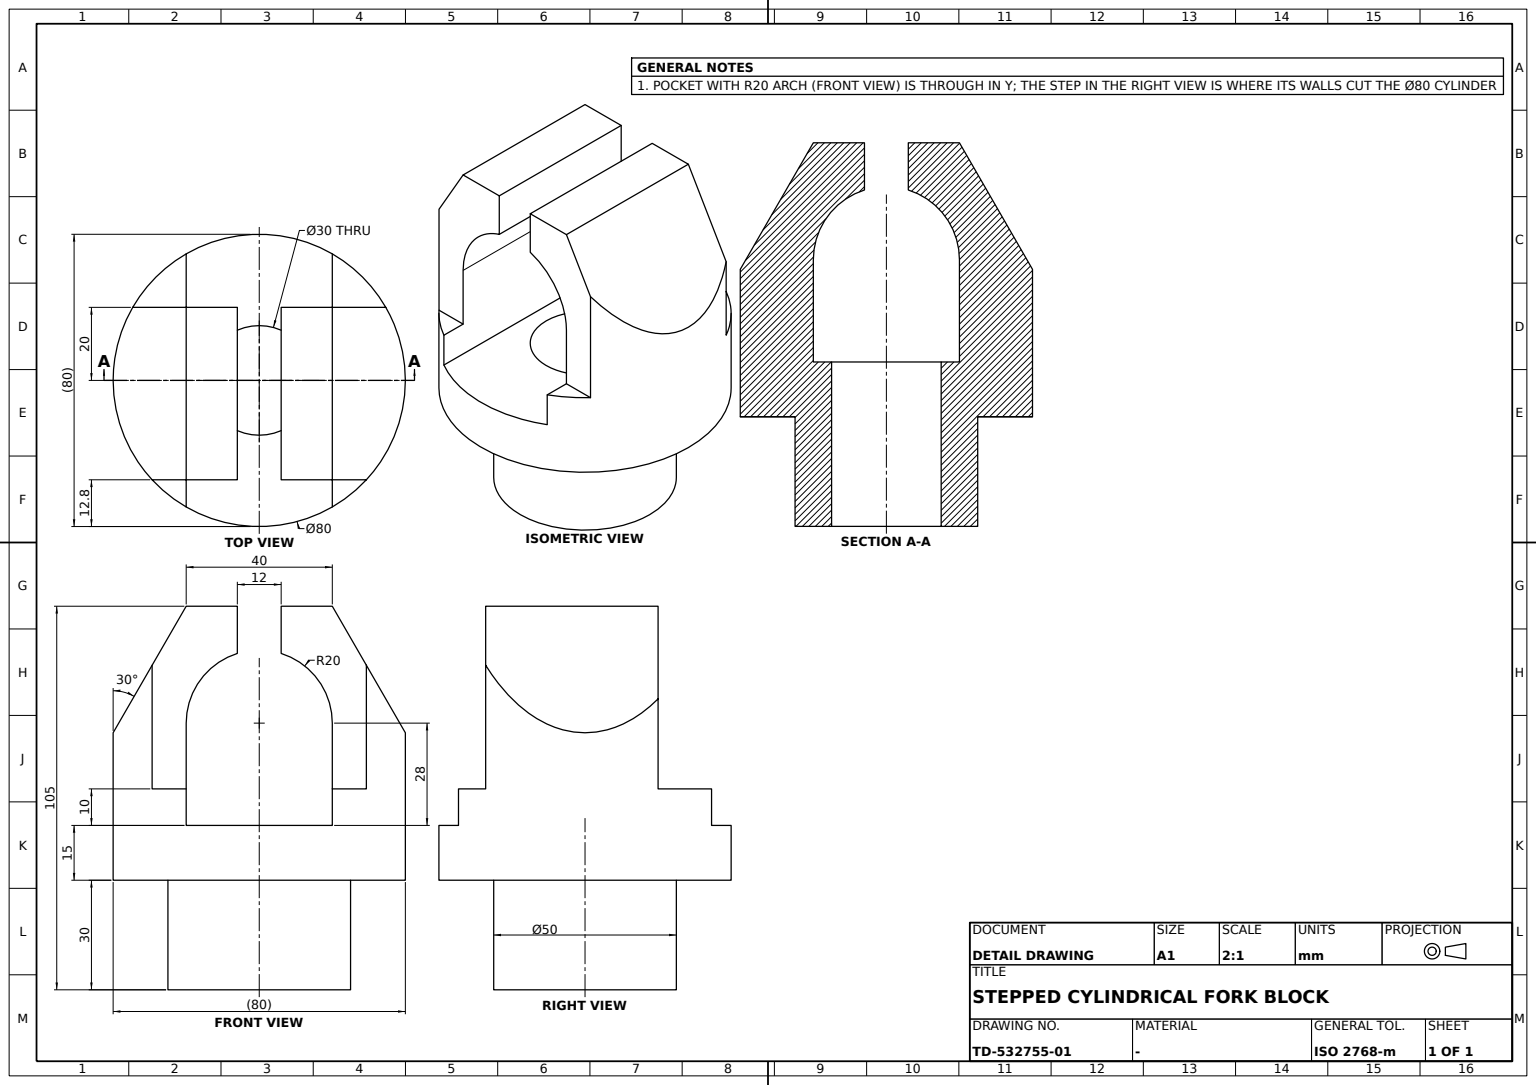
ISO-10303-21;
HEADER;
FILE_DESCRIPTION((''),'2;1');
FILE_NAME('','',(''),(''),'','','');
FILE_SCHEMA(('AUTOMOTIVE_DESIGN'));
ENDSEC;
DATA;
#1=APPLICATION_CONTEXT('');
#2=PRODUCT_CONTEXT('',#1,'mechanical');
#3=PRODUCT('','','',(#2));
#4=PRODUCT_DEFINITION_FORMATION('','',#3);
#5=PRODUCT_DEFINITION_CONTEXT('',#1,'design');
#6=PRODUCT_DEFINITION('','',#4,#5);
#7=PRODUCT_DEFINITION_SHAPE('','',#6);
#8=(LENGTH_UNIT()NAMED_UNIT(*)SI_UNIT(.MILLI.,.METRE.));
#9=(NAMED_UNIT(*)PLANE_ANGLE_UNIT()SI_UNIT($,.RADIAN.));
#10=(NAMED_UNIT(*)SI_UNIT($,.STERADIAN.)SOLID_ANGLE_UNIT());
#11=UNCERTAINTY_MEASURE_WITH_UNIT(LENGTH_MEASURE(1.E-05),#8,'distance_accuracy_value','');
#12=(GEOMETRIC_REPRESENTATION_CONTEXT(3)GLOBAL_UNCERTAINTY_ASSIGNED_CONTEXT((#11))GLOBAL_UNIT_ASSIGNED_CONTEXT((#8,#9,#10))REPRESENTATION_CONTEXT('',''));
#13=CARTESIAN_POINT('',(-6.,-27.201708,105.));
#14=VERTEX_POINT('',#13);
#15=CARTESIAN_POINT('',(-6.,-27.201708,92.078784));
#16=VERTEX_POINT('',#15);
#17=CARTESIAN_POINT('',(-6.,-27.201708,98.539392));
#18=DIRECTION('',(0.,0.,-1.));
#19=VECTOR('',#18,1000.);
#20=LINE('',#17,#19);
#21=EDGE_CURVE('',#14,#16,#20,.T.);
#22=ORIENTED_EDGE('',*,*,#21,.F.);
#23=CARTESIAN_POINT('',(-20.,-27.201708,105.));
#24=VERTEX_POINT('',#23);
#25=CARTESIAN_POINT('',(-13.,-27.201708,105.));
#26=DIRECTION('',(-1.,0.,0.));
#27=VECTOR('',#26,1000.);
#28=LINE('',#25,#27);
#29=EDGE_CURVE('',#14,#24,#28,.T.);
#30=ORIENTED_EDGE('',*,*,#29,.T.);
#31=CARTESIAN_POINT('',(-29.3269,-27.201708,88.845335));
#32=VERTEX_POINT('',#31);
#33=CARTESIAN_POINT('',(-24.66345,-27.201708,96.922667));
#34=DIRECTION('',(-0.5,0.,-0.866025404));
#35=VECTOR('',#34,1000.);
#36=LINE('',#33,#35);
#37=EDGE_CURVE('',#24,#32,#36,.T.);
#38=ORIENTED_EDGE('',*,*,#37,.T.);
#39=CARTESIAN_POINT('',(-29.3269,-27.201708,55.));
#40=VERTEX_POINT('',#39);
#41=CARTESIAN_POINT('',(-29.3269,-27.201708,71.922667));
#42=LINE('',#41,#19);
#43=EDGE_CURVE('',#32,#40,#42,.T.);
#44=ORIENTED_EDGE('',*,*,#43,.T.);
#45=CARTESIAN_POINT('',(-20.,-27.201708,55.));
#46=VERTEX_POINT('',#45);
#47=CARTESIAN_POINT('',(-24.66345,-27.201708,55.));
#48=LINE('',#47,#27);
#49=EDGE_CURVE('',#46,#40,#48,.T.);
#50=ORIENTED_EDGE('',*,*,#49,.F.);
#51=CARTESIAN_POINT('',(-20.,-27.201708,73.));
#52=VERTEX_POINT('',#51);
#53=CARTESIAN_POINT('',(-20.,-27.201708,64.));
#54=DIRECTION('',(0.,0.,1.));
#55=VECTOR('',#54,1000.);
#56=LINE('',#53,#55);
#57=EDGE_CURVE('',#46,#52,#56,.T.);
#58=ORIENTED_EDGE('',*,*,#57,.T.);
#59=CARTESIAN_POINT('',(0.,-27.201708,73.));
#60=DIRECTION('',(0.,1.,0.));
#61=AXIS2_PLACEMENT_3D('',#59,#60,#18);
#62=CIRCLE('',#61,20.);
#63=EDGE_CURVE('',#52,#16,#62,.T.);
#64=ORIENTED_EDGE('',*,*,#63,.T.);
#65=EDGE_LOOP('',(#22,#30,#38,#44,#50,#58,#64));
#66=FACE_OUTER_BOUND('',#65,.T.);
#67=CARTESIAN_POINT('',(0.,-27.201708,105.));
#68=AXIS2_PLACEMENT_3D('',#67,#60,#18);
#69=PLANE('',#68);
#70=ADVANCED_FACE('',(#66),#69,.F.);
#71=CARTESIAN_POINT('',(34.641016,20.,55.));
#72=VERTEX_POINT('',#71);
#73=CARTESIAN_POINT('',(20.,20.,55.));
#74=VERTEX_POINT('',#73);
#75=CARTESIAN_POINT('',(27.320508,20.,55.));
#76=LINE('',#75,#27);
#77=EDGE_CURVE('',#72,#74,#76,.T.);
#78=ORIENTED_EDGE('',*,*,#77,.F.);
#79=CARTESIAN_POINT('',(20.,34.641016,55.));
#80=VERTEX_POINT('',#79);
#81=CARTESIAN_POINT('',(0.,0.,55.));
#82=DIRECTION('',(0.,-1.,0.));
#83=AXIS2_PLACEMENT_3D('',#81,#18,#82);
#84=CIRCLE('',#83,40.);
#85=EDGE_CURVE('',#80,#72,#84,.T.);
#86=ORIENTED_EDGE('',*,*,#85,.F.);
#87=CARTESIAN_POINT('',(20.,27.320508,55.));
#88=VECTOR('',#82,1000.);
#89=LINE('',#87,#88);
#90=EDGE_CURVE('',#80,#74,#89,.T.);
#91=ORIENTED_EDGE('',*,*,#90,.T.);
#92=EDGE_LOOP('',(#78,#86,#91));
#93=FACE_OUTER_BOUND('',#92,.T.);
#94=CARTESIAN_POINT('',(0.,54.268078,55.));
#95=AXIS2_PLACEMENT_3D('',#94,#18,#82);
#96=PLANE('',#95);
#97=ADVANCED_FACE('',(#93),#96,.F.);
#98=CARTESIAN_POINT('',(-15.,0.,45.));
#99=VERTEX_POINT('',#98);
#100=CARTESIAN_POINT('',(15.,0.,45.));
#101=VERTEX_POINT('',#100);
#102=CARTESIAN_POINT('',(0.,0.,45.));
#103=DIRECTION('',(1.,0.,0.));
#104=AXIS2_PLACEMENT_3D('',#102,#54,#103);
#105=CIRCLE('',#104,15.);
#106=EDGE_CURVE('',#99,#101,#105,.T.);
#107=ORIENTED_EDGE('',*,*,#106,.F.);
#108=EDGE_CURVE('',#101,#99,#105,.T.);
#109=ORIENTED_EDGE('',*,*,#108,.F.);
#110=EDGE_LOOP('',(#107,#109));
#111=FACE_BOUND('',#110,.T.);
#112=CARTESIAN_POINT('',(-20.,-34.641016,45.));
#113=VERTEX_POINT('',#112);
#114=CARTESIAN_POINT('',(20.,-34.641016,45.));
#115=VERTEX_POINT('',#114);
#116=AXIS2_PLACEMENT_3D('',#102,#54,#26);
#117=CIRCLE('',#116,40.);
#118=EDGE_CURVE('',#113,#115,#117,.T.);
#119=ORIENTED_EDGE('',*,*,#118,.T.);
#120=CARTESIAN_POINT('',(20.,34.641016,45.));
#121=VERTEX_POINT('',#120);
#122=CARTESIAN_POINT('',(20.,0.,45.));
#123=LINE('',#122,#88);
#124=EDGE_CURVE('',#121,#115,#123,.T.);
#125=ORIENTED_EDGE('',*,*,#124,.F.);
#126=CARTESIAN_POINT('',(-20.,34.641016,45.));
#127=VERTEX_POINT('',#126);
#128=EDGE_CURVE('',#121,#127,#117,.T.);
#129=ORIENTED_EDGE('',*,*,#128,.T.);
#130=CARTESIAN_POINT('',(-20.,0.,45.));
#131=LINE('',#130,#88);
#132=EDGE_CURVE('',#127,#113,#131,.T.);
#133=ORIENTED_EDGE('',*,*,#132,.T.);
#134=EDGE_LOOP('',(#119,#125,#129,#133));
#135=FACE_OUTER_BOUND('',#134,.T.);
#136=AXIS2_PLACEMENT_3D('',#122,#54,#26);
#137=PLANE('',#136);
#138=ADVANCED_FACE('',(#111,#135),#137,.T.);
#139=CARTESIAN_POINT('',(-6.,20.,92.078784));
#140=VERTEX_POINT('',#139);
#141=CARTESIAN_POINT('',(-6.,-3.600854,92.078784));
#142=VECTOR('',#60,1000.);
#143=LINE('',#141,#142);
#144=EDGE_CURVE('',#16,#140,#143,.T.);
#145=ORIENTED_EDGE('',*,*,#144,.F.);
#146=ORIENTED_EDGE('',*,*,#63,.F.);
#147=CARTESIAN_POINT('',(-20.,20.,73.));
#148=VERTEX_POINT('',#147);
#149=CARTESIAN_POINT('',(-20.,-3.600854,73.));
#150=LINE('',#149,#88);
#151=EDGE_CURVE('',#148,#52,#150,.T.);
#152=ORIENTED_EDGE('',*,*,#151,.F.);
#153=CARTESIAN_POINT('',(0.,20.,73.));
#154=AXIS2_PLACEMENT_3D('',#153,#60,#18);
#155=CIRCLE('',#154,20.);
#156=EDGE_CURVE('',#148,#140,#155,.T.);
#157=ORIENTED_EDGE('',*,*,#156,.T.);
#158=EDGE_LOOP('',(#145,#146,#152,#157));
#159=FACE_OUTER_BOUND('',#158,.T.);
#160=CARTESIAN_POINT('',(0.,0.,73.));
#161=AXIS2_PLACEMENT_3D('',#160,#82,#26);
#162=CYLINDRICAL_SURFACE('',#161,20.);
#163=ADVANCED_FACE('',(#159),#162,.F.);
#164=CARTESIAN_POINT('',(-20.,20.,55.));
#165=VERTEX_POINT('',#164);
#166=CARTESIAN_POINT('',(-34.641016,20.,55.));
#167=VERTEX_POINT('',#166);
#168=CARTESIAN_POINT('',(-27.320508,20.,55.));
#169=LINE('',#168,#27);
#170=EDGE_CURVE('',#165,#167,#169,.T.);
#171=ORIENTED_EDGE('',*,*,#170,.T.);
#172=CARTESIAN_POINT('',(-34.64101,20.,79.641026));
#173=VERTEX_POINT('',#172);
#174=CARTESIAN_POINT('',(-34.641016,20.,67.320515));
#175=LINE('',#174,#19);
#176=EDGE_CURVE('',#173,#167,#175,.T.);
#177=ORIENTED_EDGE('',*,*,#176,.F.);
#178=CARTESIAN_POINT('',(-20.,20.,105.));
#179=VERTEX_POINT('',#178);
#180=CARTESIAN_POINT('',(-27.320505,20.,92.320513));
#181=LINE('',#180,#35);
#182=EDGE_CURVE('',#179,#173,#181,.T.);
#183=ORIENTED_EDGE('',*,*,#182,.F.);
#184=CARTESIAN_POINT('',(-6.,20.,105.));
#185=VERTEX_POINT('',#184);
#186=CARTESIAN_POINT('',(-13.,20.,105.));
#187=LINE('',#186,#27);
#188=EDGE_CURVE('',#185,#179,#187,.T.);
#189=ORIENTED_EDGE('',*,*,#188,.F.);
#190=CARTESIAN_POINT('',(-6.,20.,98.539392));
#191=LINE('',#190,#19);
#192=EDGE_CURVE('',#185,#140,#191,.T.);
#193=ORIENTED_EDGE('',*,*,#192,.T.);
#194=ORIENTED_EDGE('',*,*,#156,.F.);
#195=CARTESIAN_POINT('',(-20.,20.,64.));
#196=LINE('',#195,#55);
#197=EDGE_CURVE('',#165,#148,#196,.T.);
#198=ORIENTED_EDGE('',*,*,#197,.F.);
#199=EDGE_LOOP('',(#171,#177,#183,#189,#193,#194,#198));
#200=FACE_OUTER_BOUND('',#199,.T.);
#201=CARTESIAN_POINT('',(0.,20.,105.));
#202=AXIS2_PLACEMENT_3D('',#201,#60,#18);
#203=PLANE('',#202);
#204=ADVANCED_FACE('',(#200),#203,.T.);
#205=ORIENTED_EDGE('',*,*,#176,.T.);
#206=CARTESIAN_POINT('',(-20.,34.641016,55.));
#207=VERTEX_POINT('',#206);
#208=EDGE_CURVE('',#167,#207,#84,.T.);
#209=ORIENTED_EDGE('',*,*,#208,.T.);
#210=CARTESIAN_POINT('',(-20.,34.641016,50.));
#211=LINE('',#210,#19);
#212=EDGE_CURVE('',#207,#127,#211,.T.);
#213=ORIENTED_EDGE('',*,*,#212,.T.);
#214=ORIENTED_EDGE('',*,*,#128,.F.);
#215=CARTESIAN_POINT('',(20.,34.641016,50.));
#216=LINE('',#215,#19);
#217=EDGE_CURVE('',#80,#121,#216,.T.);
#218=ORIENTED_EDGE('',*,*,#217,.F.);
#219=ORIENTED_EDGE('',*,*,#85,.T.);
#220=CARTESIAN_POINT('',(34.641014,20.,79.64102));
#221=VERTEX_POINT('',#220);
#222=CARTESIAN_POINT('',(34.641016,20.,67.320513));
#223=LINE('',#222,#19);
#224=EDGE_CURVE('',#221,#72,#223,.T.);
#225=ORIENTED_EDGE('',*,*,#224,.F.);
#226=CARTESIAN_POINT('',(40.,0.,70.358984));
#227=VERTEX_POINT('',#226);
#228=CARTESIAN_POINT('',(40.,1.413947,70.358984));
#229=CARTESIAN_POINT('',(39.937524,2.827895,70.467196));
#230=CARTESIAN_POINT('',(39.812558,4.226252,70.683644));
#231=CARTESIAN_POINT('',(39.408602,7.253337,71.383316));
#232=CARTESIAN_POINT('',(38.751916,10.102583,72.520729));
#233=CARTESIAN_POINT('',(38.327142,11.596307,73.256459));
#234=CARTESIAN_POINT('',(37.414843,14.315753,74.836608));
#235=CARTESIAN_POINT('',(36.340749,16.785996,76.696993));
#236=CARTESIAN_POINT('',(35.798175,17.908924,77.636759));
#237=CARTESIAN_POINT('',(35.230298,18.979329,78.62035));
#238=B_SPLINE_CURVE_WITH_KNOTS('',5,(#226,#228,#229,#230,#231,#232,#233,#234,#235,#236,#237,#220),.UNSPECIFIED.,.F.,.F.,(6,3,3,6),(0.,9.998118497,22.08747895,33.105354258),.UNSPECIFIED.);
#239=EDGE_CURVE('',#227,#221,#238,.T.);
#240=ORIENTED_EDGE('',*,*,#239,.F.);
#241=CARTESIAN_POINT('',(40.,0.,30.));
#242=VERTEX_POINT('',#241);
#243=CARTESIAN_POINT('',(40.,0.,67.5));
#244=LINE('',#243,#55);
#245=EDGE_CURVE('',#242,#227,#244,.T.);
#246=ORIENTED_EDGE('',*,*,#245,.F.);
#247=CARTESIAN_POINT('',(-40.,0.,30.));
#248=VERTEX_POINT('',#247);
#249=CARTESIAN_POINT('',(0.,0.,30.));
#250=AXIS2_PLACEMENT_3D('',#249,#54,#103);
#251=CIRCLE('',#250,40.);
#252=EDGE_CURVE('',#242,#248,#251,.T.);
#253=ORIENTED_EDGE('',*,*,#252,.T.);
#254=CARTESIAN_POINT('',(-40.,0.,70.358984));
#255=VERTEX_POINT('',#254);
#256=CARTESIAN_POINT('',(-40.,0.,67.5));
#257=LINE('',#256,#55);
#258=EDGE_CURVE('',#248,#255,#257,.T.);
#259=ORIENTED_EDGE('',*,*,#258,.T.);
#260=CARTESIAN_POINT('',(-35.357637,18.758763,78.399792));
#261=CARTESIAN_POINT('',(-36.04274,17.443742,77.213159));
#262=CARTESIAN_POINT('',(-36.689164,16.050084,76.093519));
#263=CARTESIAN_POINT('',(-37.760649,13.404531,74.237654));
#264=CARTESIAN_POINT('',(-38.636028,10.48908,72.721453));
#265=CARTESIAN_POINT('',(-38.9784,9.146917,72.128448));
#266=CARTESIAN_POINT('',(-39.5153,6.564102,71.198509));
#267=CARTESIAN_POINT('',(-39.844785,3.848374,70.627824));
#268=CARTESIAN_POINT('',(-39.948262,2.573371,70.448597));
#269=CARTESIAN_POINT('',(-40.,1.286704,70.358984));
#270=B_SPLINE_CURVE_WITH_KNOTS('',5,(#172,#260,#261,#262,#263,#264,#265,#266,#267,#268,#269,#254),.UNSPECIFIED.,.F.,.F.,(6,3,3,6),(46.642174313,60.032180899,70.642912035,79.741294563),.UNSPECIFIED.);
#271=EDGE_CURVE('',#173,#255,#270,.T.);
#272=ORIENTED_EDGE('',*,*,#271,.F.);
#273=EDGE_LOOP('',(#205,#209,#213,#214,#218,#219,#225,#240,#246,#253,#259,#272));
#274=FACE_OUTER_BOUND('',#273,.T.);
#275=CARTESIAN_POINT('',(0.,0.,67.5));
#276=AXIS2_PLACEMENT_3D('',#275,#18,#103);
#277=CYLINDRICAL_SURFACE('',#276,40.);
#278=ADVANCED_FACE('',(#274),#277,.T.);
#279=CARTESIAN_POINT('',(20.,20.,73.));
#280=VERTEX_POINT('',#279);
#281=CARTESIAN_POINT('',(20.,-27.201708,73.));
#282=VERTEX_POINT('',#281);
#283=CARTESIAN_POINT('',(20.,-3.600854,73.));
#284=LINE('',#283,#88);
#285=EDGE_CURVE('',#280,#282,#284,.T.);
#286=ORIENTED_EDGE('',*,*,#285,.T.);
#287=CARTESIAN_POINT('',(6.,-27.201708,92.078784));
#288=VERTEX_POINT('',#287);
#289=EDGE_CURVE('',#288,#282,#62,.T.);
#290=ORIENTED_EDGE('',*,*,#289,.F.);
#291=CARTESIAN_POINT('',(6.,20.,92.078784));
#292=VERTEX_POINT('',#291);
#293=CARTESIAN_POINT('',(6.,-3.600854,92.078784));
#294=LINE('',#293,#88);
#295=EDGE_CURVE('',#292,#288,#294,.T.);
#296=ORIENTED_EDGE('',*,*,#295,.F.);
#297=EDGE_CURVE('',#292,#280,#155,.T.);
#298=ORIENTED_EDGE('',*,*,#297,.T.);
#299=EDGE_LOOP('',(#286,#290,#296,#298));
#300=FACE_OUTER_BOUND('',#299,.T.);
#301=ADVANCED_FACE('',(#300),#162,.F.);
#302=ORIENTED_EDGE('',*,*,#208,.F.);
#303=ORIENTED_EDGE('',*,*,#170,.F.);
#304=CARTESIAN_POINT('',(-20.,27.320508,55.));
#305=LINE('',#304,#88);
#306=EDGE_CURVE('',#207,#165,#305,.T.);
#307=ORIENTED_EDGE('',*,*,#306,.F.);
#308=EDGE_LOOP('',(#302,#303,#307));
#309=FACE_OUTER_BOUND('',#308,.T.);
#310=ADVANCED_FACE('',(#309),#96,.F.);
#311=CARTESIAN_POINT('',(-25.,0.,0.));
#312=VERTEX_POINT('',#311);
#313=CARTESIAN_POINT('',(-25.,0.,30.));
#314=VERTEX_POINT('',#313);
#315=CARTESIAN_POINT('',(-25.,0.,15.));
#316=LINE('',#315,#55);
#317=EDGE_CURVE('',#312,#314,#316,.T.);
#318=ORIENTED_EDGE('',*,*,#317,.F.);
#319=CARTESIAN_POINT('',(25.,0.,0.));
#320=VERTEX_POINT('',#319);
#321=CARTESIAN_POINT('',(0.,0.,0.));
#322=AXIS2_PLACEMENT_3D('',#321,#54,#103);
#323=CIRCLE('',#322,25.);
#324=EDGE_CURVE('',#312,#320,#323,.T.);
#325=ORIENTED_EDGE('',*,*,#324,.T.);
#326=CARTESIAN_POINT('',(25.,0.,30.));
#327=VERTEX_POINT('',#326);
#328=CARTESIAN_POINT('',(25.,0.,15.));
#329=LINE('',#328,#55);
#330=EDGE_CURVE('',#320,#327,#329,.T.);
#331=ORIENTED_EDGE('',*,*,#330,.T.);
#332=CIRCLE('',#250,25.);
#333=EDGE_CURVE('',#314,#327,#332,.T.);
#334=ORIENTED_EDGE('',*,*,#333,.F.);
#335=EDGE_LOOP('',(#318,#325,#331,#334));
#336=FACE_OUTER_BOUND('',#335,.T.);
#337=CARTESIAN_POINT('',(0.,0.,15.));
#338=AXIS2_PLACEMENT_3D('',#337,#18,#103);
#339=CYLINDRICAL_SURFACE('',#338,25.);
#340=ADVANCED_FACE('',(#336),#339,.T.);
#341=CARTESIAN_POINT('',(20.,-27.201708,105.));
#342=VERTEX_POINT('',#341);
#343=CARTESIAN_POINT('',(29.326899,-27.201709,88.845336));
#344=VERTEX_POINT('',#343);
#345=CARTESIAN_POINT('',(24.66345,-27.201708,96.922667));
#346=DIRECTION('',(0.5,0.,-0.866025404));
#347=VECTOR('',#346,1000.);
#348=LINE('',#345,#347);
#349=EDGE_CURVE('',#342,#344,#348,.T.);
#350=ORIENTED_EDGE('',*,*,#349,.T.);
#351=CARTESIAN_POINT('',(40.,-1.413947,70.358984));
#352=CARTESIAN_POINT('',(39.937524,-2.827895,70.467196));
#353=CARTESIAN_POINT('',(39.812558,-4.226252,70.683644));
#354=CARTESIAN_POINT('',(39.408602,-7.253337,71.383316));
#355=CARTESIAN_POINT('',(38.751916,-10.102583,72.520729));
#356=CARTESIAN_POINT('',(38.327142,-11.596307,73.256459));
#357=CARTESIAN_POINT('',(37.089655,-15.285096,75.39985));
#358=CARTESIAN_POINT('',(35.554474,-18.515363,78.058862));
#359=CARTESIAN_POINT('',(34.532988,-20.335945,79.828126));
#360=CARTESIAN_POINT('',(32.898568,-22.872681,82.659025));
#361=CARTESIAN_POINT('',(31.160566,-25.107645,85.669333));
#362=CARTESIAN_POINT('',(30.557999,-25.836287,86.713009));
#363=CARTESIAN_POINT('',(29.946433,-26.533773,87.772273));
#364=B_SPLINE_CURVE_WITH_KNOTS('',5,(#226,#351,#352,#353,#354,#355,#356,#357,#358,#359,#360,#361,#362,#363,#343),.UNSPECIFIED.,.F.,.F.,(6,3,3,3,6),(0.,9.9981185,22.087478954,41.34189657,51.295457243),.UNSPECIFIED.);
#365=EDGE_CURVE('',#227,#344,#364,.T.);
#366=ORIENTED_EDGE('',*,*,#365,.F.);
#367=ORIENTED_EDGE('',*,*,#239,.T.);
#368=CARTESIAN_POINT('',(20.,20.,105.));
#369=VERTEX_POINT('',#368);
#370=CARTESIAN_POINT('',(27.320507,20.,92.32051));
#371=LINE('',#370,#347);
#372=EDGE_CURVE('',#369,#221,#371,.T.);
#373=ORIENTED_EDGE('',*,*,#372,.F.);
#374=CARTESIAN_POINT('',(20.,-3.600854,105.));
#375=LINE('',#374,#88);
#376=EDGE_CURVE('',#369,#342,#375,.T.);
#377=ORIENTED_EDGE('',*,*,#376,.T.);
#378=EDGE_LOOP('',(#350,#366,#367,#373,#377));
#379=FACE_OUTER_BOUND('',#378,.T.);
#380=CARTESIAN_POINT('',(49.937466,0.,53.146788));
#381=DIRECTION('',(0.866025404,0.,0.5));
#382=DIRECTION('',(-0.5,0.,0.866025404));
#383=AXIS2_PLACEMENT_3D('',#380,#381,#382);
#384=PLANE('',#383);
#385=ADVANCED_FACE('',(#379),#384,.T.);
#386=ORIENTED_EDGE('',*,*,#330,.F.);
#387=EDGE_CURVE('',#320,#312,#323,.T.);
#388=ORIENTED_EDGE('',*,*,#387,.T.);
#389=ORIENTED_EDGE('',*,*,#317,.T.);
#390=EDGE_CURVE('',#327,#314,#332,.T.);
#391=ORIENTED_EDGE('',*,*,#390,.F.);
#392=EDGE_LOOP('',(#386,#388,#389,#391));
#393=FACE_OUTER_BOUND('',#392,.T.);
#394=ADVANCED_FACE('',(#393),#339,.T.);
#395=ORIENTED_EDGE('',*,*,#372,.T.);
#396=ORIENTED_EDGE('',*,*,#224,.T.);
#397=ORIENTED_EDGE('',*,*,#77,.T.);
#398=CARTESIAN_POINT('',(20.,20.,64.));
#399=LINE('',#398,#55);
#400=EDGE_CURVE('',#74,#280,#399,.T.);
#401=ORIENTED_EDGE('',*,*,#400,.T.);
#402=ORIENTED_EDGE('',*,*,#297,.F.);
#403=CARTESIAN_POINT('',(6.,20.,105.));
#404=VERTEX_POINT('',#403);
#405=CARTESIAN_POINT('',(6.,20.,98.539392));
#406=LINE('',#405,#19);
#407=EDGE_CURVE('',#404,#292,#406,.T.);
#408=ORIENTED_EDGE('',*,*,#407,.F.);
#409=CARTESIAN_POINT('',(13.,20.,105.));
#410=LINE('',#409,#27);
#411=EDGE_CURVE('',#369,#404,#410,.T.);
#412=ORIENTED_EDGE('',*,*,#411,.F.);
#413=EDGE_LOOP('',(#395,#396,#397,#401,#402,#408,#412));
#414=FACE_OUTER_BOUND('',#413,.T.);
#415=ADVANCED_FACE('',(#414),#203,.T.);
#416=CARTESIAN_POINT('',(-20.,-3.600854,105.));
#417=LINE('',#416,#88);
#418=EDGE_CURVE('',#179,#24,#417,.T.);
#419=ORIENTED_EDGE('',*,*,#418,.T.);
#420=ORIENTED_EDGE('',*,*,#29,.F.);
#421=CARTESIAN_POINT('',(-6.,-3.600854,105.));
#422=LINE('',#421,#88);
#423=EDGE_CURVE('',#185,#14,#422,.T.);
#424=ORIENTED_EDGE('',*,*,#423,.F.);
#425=ORIENTED_EDGE('',*,*,#188,.T.);
#426=EDGE_LOOP('',(#419,#420,#424,#425));
#427=FACE_OUTER_BOUND('',#426,.T.);
#428=CARTESIAN_POINT('',(0.,0.,105.));
#429=AXIS2_PLACEMENT_3D('',#428,#54,#103);
#430=PLANE('',#429);
#431=ADVANCED_FACE('',(#427),#430,.T.);
#432=ORIENTED_EDGE('',*,*,#106,.T.);
#433=CARTESIAN_POINT('',(15.,0.,0.));
#434=VERTEX_POINT('',#433);
#435=CARTESIAN_POINT('',(15.,0.,21.84));
#436=LINE('',#435,#19);
#437=EDGE_CURVE('',#101,#434,#436,.T.);
#438=ORIENTED_EDGE('',*,*,#437,.T.);
#439=CARTESIAN_POINT('',(-15.,0.,0.));
#440=VERTEX_POINT('',#439);
#441=CIRCLE('',#322,15.);
#442=EDGE_CURVE('',#440,#434,#441,.T.);
#443=ORIENTED_EDGE('',*,*,#442,.F.);
#444=CARTESIAN_POINT('',(-15.,0.,21.84));
#445=LINE('',#444,#19);
#446=EDGE_CURVE('',#99,#440,#445,.T.);
#447=ORIENTED_EDGE('',*,*,#446,.F.);
#448=EDGE_LOOP('',(#432,#438,#443,#447));
#449=FACE_OUTER_BOUND('',#448,.T.);
#450=CARTESIAN_POINT('',(0.,0.,21.84));
#451=AXIS2_PLACEMENT_3D('',#450,#18,#103);
#452=CYLINDRICAL_SURFACE('',#451,15.);
#453=ADVANCED_FACE('',(#449),#452,.F.);
#454=CARTESIAN_POINT('',(20.,-27.201708,55.));
#455=VERTEX_POINT('',#454);
#456=CARTESIAN_POINT('',(20.,-34.641016,55.));
#457=VERTEX_POINT('',#456);
#458=CARTESIAN_POINT('',(20.,-30.921362,55.));
#459=LINE('',#458,#88);
#460=EDGE_CURVE('',#455,#457,#459,.T.);
#461=ORIENTED_EDGE('',*,*,#460,.T.);
#462=CARTESIAN_POINT('',(29.3269,-27.201708,55.));
#463=VERTEX_POINT('',#462);
#464=EDGE_CURVE('',#463,#457,#84,.T.);
#465=ORIENTED_EDGE('',*,*,#464,.F.);
#466=CARTESIAN_POINT('',(24.66345,-27.201708,55.));
#467=LINE('',#466,#27);
#468=EDGE_CURVE('',#463,#455,#467,.T.);
#469=ORIENTED_EDGE('',*,*,#468,.T.);
#470=EDGE_LOOP('',(#461,#465,#469));
#471=FACE_OUTER_BOUND('',#470,.T.);
#472=ADVANCED_FACE('',(#471),#96,.F.);
#473=CARTESIAN_POINT('',(-20.,-34.641016,55.));
#474=VERTEX_POINT('',#473);
#475=CARTESIAN_POINT('',(-20.,-30.921362,55.));
#476=LINE('',#475,#88);
#477=EDGE_CURVE('',#46,#474,#476,.T.);
#478=ORIENTED_EDGE('',*,*,#477,.F.);
#479=ORIENTED_EDGE('',*,*,#49,.T.);
#480=EDGE_CURVE('',#474,#40,#84,.T.);
#481=ORIENTED_EDGE('',*,*,#480,.F.);
#482=EDGE_LOOP('',(#478,#479,#481));
#483=FACE_OUTER_BOUND('',#482,.T.);
#484=ADVANCED_FACE('',(#483),#96,.F.);
#485=ORIENTED_EDGE('',*,*,#324,.F.);
#486=ORIENTED_EDGE('',*,*,#387,.F.);
#487=EDGE_LOOP('',(#485,#486));
#488=FACE_OUTER_BOUND('',#487,.T.);
#489=EDGE_CURVE('',#434,#440,#441,.T.);
#490=ORIENTED_EDGE('',*,*,#489,.T.);
#491=ORIENTED_EDGE('',*,*,#442,.T.);
#492=EDGE_LOOP('',(#490,#491));
#493=FACE_BOUND('',#492,.T.);
#494=PLANE('',#322);
#495=ADVANCED_FACE('',(#488,#493),#494,.F.);
#496=ORIENTED_EDGE('',*,*,#423,.T.);
#497=ORIENTED_EDGE('',*,*,#21,.T.);
#498=ORIENTED_EDGE('',*,*,#144,.T.);
#499=ORIENTED_EDGE('',*,*,#192,.F.);
#500=EDGE_LOOP('',(#496,#497,#498,#499));
#501=FACE_OUTER_BOUND('',#500,.T.);
#502=CARTESIAN_POINT('',(-6.,-55.080074,105.));
#503=AXIS2_PLACEMENT_3D('',#502,#26,#60);
#504=PLANE('',#503);
#505=ADVANCED_FACE('',(#501),#504,.F.);
#506=ORIENTED_EDGE('',*,*,#271,.T.);
#507=CARTESIAN_POINT('',(-40.,-0.027618,70.358984));
#508=CARTESIAN_POINT('',(-39.999976,-0.055235,70.359025));
#509=CARTESIAN_POINT('',(-39.999928,-0.082853,70.359108));
#510=CARTESIAN_POINT('',(-39.995847,-1.659413,70.366178));
#511=CARTESIAN_POINT('',(-39.914096,-3.234899,70.507775));
#512=CARTESIAN_POINT('',(-39.759005,-4.761191,70.776399));
#513=CARTESIAN_POINT('',(-39.28551,-7.922627,71.596516));
#514=CARTESIAN_POINT('',(-38.543227,-10.873373,72.882188));
#515=CARTESIAN_POINT('',(-38.086553,-12.364558,73.673172));
#516=CARTESIAN_POINT('',(-36.948255,-15.542958,75.644761));
#517=CARTESIAN_POINT('',(-35.594352,-18.368981,77.98979));
#518=CARTESIAN_POINT('',(-34.794215,-19.831861,79.375668));
#519=CARTESIAN_POINT('',(-33.266209,-22.323678,82.022252));
#520=CARTESIAN_POINT('',(-31.632513,-24.528234,84.851897));
#521=CARTESIAN_POINT('',(-30.878057,-25.46861,86.158652));
#522=CARTESIAN_POINT('',(-30.108824,-26.358695,87.491003));
#523=B_SPLINE_CURVE_WITH_KNOTS('',5,(#254,#507,#508,#509,#510,#511,#512,#513,#514,#515,#516,#517,#518,#519,#520,#521,#522,#31),.UNSPECIFIED.,.F.,.F.,(6,3,3,3,3,6),(79.741294563,79.936581357,90.889386708,103.193331802,118.478727335,131.041165045),.UNSPECIFIED.);
#524=EDGE_CURVE('',#255,#32,#523,.T.);
#525=ORIENTED_EDGE('',*,*,#524,.T.);
#526=ORIENTED_EDGE('',*,*,#37,.F.);
#527=ORIENTED_EDGE('',*,*,#418,.F.);
#528=ORIENTED_EDGE('',*,*,#182,.T.);
#529=EDGE_LOOP('',(#506,#525,#526,#527,#528));
#530=FACE_OUTER_BOUND('',#529,.T.);
#531=CARTESIAN_POINT('',(-20.,0.,105.));
#532=DIRECTION('',(-0.866025404,0.,0.5));
#533=AXIS2_PLACEMENT_3D('',#531,#532,#34);
#534=PLANE('',#533);
#535=ADVANCED_FACE('',(#530),#534,.T.);
#536=CARTESIAN_POINT('',(6.,-27.201708,105.));
#537=VERTEX_POINT('',#536);
#538=CARTESIAN_POINT('',(6.,-27.201708,98.539392));
#539=LINE('',#538,#19);
#540=EDGE_CURVE('',#537,#288,#539,.T.);
#541=ORIENTED_EDGE('',*,*,#540,.F.);
#542=CARTESIAN_POINT('',(6.,-3.600854,105.));
#543=LINE('',#542,#142);
#544=EDGE_CURVE('',#537,#404,#543,.T.);
#545=ORIENTED_EDGE('',*,*,#544,.T.);
#546=ORIENTED_EDGE('',*,*,#407,.T.);
#547=ORIENTED_EDGE('',*,*,#295,.T.);
#548=EDGE_LOOP('',(#541,#545,#546,#547));
#549=FACE_OUTER_BOUND('',#548,.T.);
#550=CARTESIAN_POINT('',(6.,55.080074,105.));
#551=AXIS2_PLACEMENT_3D('',#550,#103,#82);
#552=PLANE('',#551);
#553=ADVANCED_FACE('',(#549),#552,.F.);
#554=ORIENTED_EDGE('',*,*,#197,.T.);
#555=ORIENTED_EDGE('',*,*,#151,.T.);
#556=ORIENTED_EDGE('',*,*,#57,.F.);
#557=ORIENTED_EDGE('',*,*,#477,.T.);
#558=CARTESIAN_POINT('',(-20.,-34.641016,50.));
#559=LINE('',#558,#19);
#560=EDGE_CURVE('',#474,#113,#559,.T.);
#561=ORIENTED_EDGE('',*,*,#560,.T.);
#562=ORIENTED_EDGE('',*,*,#132,.F.);
#563=ORIENTED_EDGE('',*,*,#212,.F.);
#564=ORIENTED_EDGE('',*,*,#306,.T.);
#565=EDGE_LOOP('',(#554,#555,#556,#557,#561,#562,#563,#564));
#566=FACE_OUTER_BOUND('',#565,.T.);
#567=CARTESIAN_POINT('',(-20.,0.,73.));
#568=AXIS2_PLACEMENT_3D('',#567,#26,#18);
#569=PLANE('',#568);
#570=ADVANCED_FACE('',(#566),#569,.F.);
#571=ORIENTED_EDGE('',*,*,#544,.F.);
#572=CARTESIAN_POINT('',(13.,-27.201708,105.));
#573=LINE('',#572,#27);
#574=EDGE_CURVE('',#342,#537,#573,.T.);
#575=ORIENTED_EDGE('',*,*,#574,.F.);
#576=ORIENTED_EDGE('',*,*,#376,.F.);
#577=ORIENTED_EDGE('',*,*,#411,.T.);
#578=EDGE_LOOP('',(#571,#575,#576,#577));
#579=FACE_OUTER_BOUND('',#578,.T.);
#580=ADVANCED_FACE('',(#579),#430,.T.);
#581=ORIENTED_EDGE('',*,*,#480,.T.);
#582=ORIENTED_EDGE('',*,*,#43,.F.);
#583=ORIENTED_EDGE('',*,*,#524,.F.);
#584=ORIENTED_EDGE('',*,*,#258,.F.);
#585=EDGE_CURVE('',#248,#242,#251,.T.);
#586=ORIENTED_EDGE('',*,*,#585,.T.);
#587=ORIENTED_EDGE('',*,*,#245,.T.);
#588=ORIENTED_EDGE('',*,*,#365,.T.);
#589=CARTESIAN_POINT('',(29.3269,-27.201708,71.922668));
#590=LINE('',#589,#19);
#591=EDGE_CURVE('',#344,#463,#590,.T.);
#592=ORIENTED_EDGE('',*,*,#591,.T.);
#593=ORIENTED_EDGE('',*,*,#464,.T.);
#594=CARTESIAN_POINT('',(20.,-34.641016,50.));
#595=LINE('',#594,#19);
#596=EDGE_CURVE('',#457,#115,#595,.T.);
#597=ORIENTED_EDGE('',*,*,#596,.T.);
#598=ORIENTED_EDGE('',*,*,#118,.F.);
#599=ORIENTED_EDGE('',*,*,#560,.F.);
#600=EDGE_LOOP('',(#581,#582,#583,#584,#586,#587,#588,#592,#593,#597,#598,#599));
#601=FACE_OUTER_BOUND('',#600,.T.);
#602=ADVANCED_FACE('',(#601),#277,.T.);
#603=ORIENTED_EDGE('',*,*,#390,.T.);
#604=ORIENTED_EDGE('',*,*,#333,.T.);
#605=EDGE_LOOP('',(#603,#604));
#606=FACE_BOUND('',#605,.T.);
#607=ORIENTED_EDGE('',*,*,#585,.F.);
#608=ORIENTED_EDGE('',*,*,#252,.F.);
#609=EDGE_LOOP('',(#607,#608));
#610=FACE_OUTER_BOUND('',#609,.T.);
#611=PLANE('',#250);
#612=ADVANCED_FACE('',(#606,#610),#611,.F.);
#613=CARTESIAN_POINT('',(20.,-27.201708,64.));
#614=LINE('',#613,#55);
#615=EDGE_CURVE('',#455,#282,#614,.T.);
#616=ORIENTED_EDGE('',*,*,#615,.T.);
#617=ORIENTED_EDGE('',*,*,#285,.F.);
#618=ORIENTED_EDGE('',*,*,#400,.F.);
#619=ORIENTED_EDGE('',*,*,#90,.F.);
#620=ORIENTED_EDGE('',*,*,#217,.T.);
#621=ORIENTED_EDGE('',*,*,#124,.T.);
#622=ORIENTED_EDGE('',*,*,#596,.F.);
#623=ORIENTED_EDGE('',*,*,#460,.F.);
#624=EDGE_LOOP('',(#616,#617,#618,#619,#620,#621,#622,#623));
#625=FACE_OUTER_BOUND('',#624,.T.);
#626=CARTESIAN_POINT('',(20.,0.,73.));
#627=AXIS2_PLACEMENT_3D('',#626,#26,#18);
#628=PLANE('',#627);
#629=ADVANCED_FACE('',(#625),#628,.T.);
#630=ORIENTED_EDGE('',*,*,#489,.F.);
#631=ORIENTED_EDGE('',*,*,#437,.F.);
#632=ORIENTED_EDGE('',*,*,#108,.T.);
#633=ORIENTED_EDGE('',*,*,#446,.T.);
#634=EDGE_LOOP('',(#630,#631,#632,#633));
#635=FACE_OUTER_BOUND('',#634,.T.);
#636=ADVANCED_FACE('',(#635),#452,.F.);
#637=ORIENTED_EDGE('',*,*,#574,.T.);
#638=ORIENTED_EDGE('',*,*,#540,.T.);
#639=ORIENTED_EDGE('',*,*,#289,.T.);
#640=ORIENTED_EDGE('',*,*,#615,.F.);
#641=ORIENTED_EDGE('',*,*,#468,.F.);
#642=ORIENTED_EDGE('',*,*,#591,.F.);
#643=ORIENTED_EDGE('',*,*,#349,.F.);
#644=EDGE_LOOP('',(#637,#638,#639,#640,#641,#642,#643));
#645=FACE_OUTER_BOUND('',#644,.T.);
#646=ADVANCED_FACE('',(#645),#69,.F.);
#647=CLOSED_SHELL('',(#70,#97,#138,#163,#204,#278,#301,#310,#340,#385,#394,#415,#431,#453,#472,#484,#495,#505,#535,#553,#570,#580,#602,#612,#629,#636,#646));
#648=MANIFOLD_SOLID_BREP('',#647);
#649=ADVANCED_BREP_SHAPE_REPRESENTATION('',(#648),#12);
#650=SHAPE_DEFINITION_REPRESENTATION(#7,#649);
ENDSEC;
END-ISO-10303-21;
